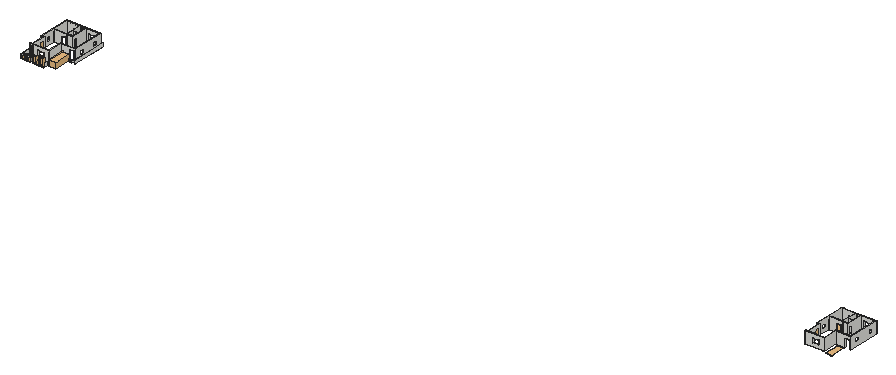
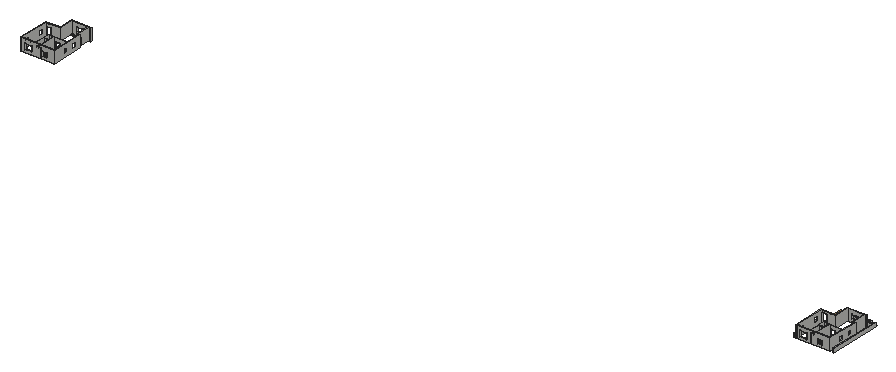
# SketchUp Ruby script. Lengths in inches.
U = 1.inch
M = Sketchup.active_model
def pt(a) = Geom::Point3d.new(a.map { |v| v * U })
def face(e, loops, mat)
  f = e.add_face(loops[0].map { |a| pt(a) })
  loops[1..].each { |l| e.add_face(l.map { |a| pt(a) }).erase! }
  f.material = f.back_material = mat if mat
  f
end
# faces: each face lists its corners as indices into pts; further lists are holes
def faces(e, pts, list, mat = nil) = list.each { |f| face(e, (f[0].is_a?(Array) ? f : [f]).map { |l| l.map { |i| pts[i] } }, mat) }
# xy, xz, yz: faces in a plane at the given z, y or x. An outline is a flat list of corners, or four numbers for a rectangle; further outlines are holes
def ring(l) = l.size == 4 ? [[l[0], l[1]], [l[2], l[1]], [l[2], l[3]], [l[0], l[3]]] : l.each_slice(2).to_a
def flat(e, list, mat, &to3) = list.each { |f| face(e, (f[0].is_a?(Array) ? f : [f]).map { |l| ring(l).map { |u, v| to3.(u, v) } }, mat) }
def xy(e, z, list, mat = nil) = flat(e, list, mat) { |x, y| [x, y, z] }
def xz(e, y, list, mat = nil) = flat(e, list, mat) { |x, z| [x, y, z] }
def yz(e, x, list, mat = nil) = flat(e, list, mat) { |y, z| [x, y, z] }
def lines(e, pts, list) = list.each { |a, b| e.add_line(pt(pts[a]), pt(pts[b])) }
# prism: a flat outline (further loops are holes) pulled along v
def prism(e, loops, v, mat = nil)
  f = face(e, loops, mat); d = Geom::Vector3d.new(v.map { |x| x * U })
  f.pushpull(f.normal.samedirection?(d) ? d.length : -d.length)
end
def box(e, o, s, mat = nil) = prism(e, [[o, [o[0] + s[0], o[1], o[2]], [o[0] + s[0], o[1] + s[1], o[2]], [o[0], o[1] + s[1], o[2]]]], [0, 0, s[2]], mat)
def at(x, y, z, deg = 0) = Geom::Transformation.translation(pt([x, y, z])) * Geom::Transformation.rotation(ORIGIN, Z_AXIS, deg.degrees)
def axes(o, x, y, z) = Geom::Transformation.new([*x, 0, *y, 0, *z, 0, *pt(o).to_a, 1])
def part(name) = M.definitions.add(name)
# library, detail: a bought-in or finely detailed component or shape, given as its bounding box
def library(name, o, s) = part(name).tap { |d| box(d.entities, o, s) }
def detail(e, o, s) = box(e.add_group.entities, o, s)
def put(e, d, t, mat = nil) = e.add_instance(d, t).tap { |i| i.material = mat if mat }
def group(e, t, mat = nil) = e.add_group.tap { |g| g.transformation = t; g.material = mat if mat }.entities
root = M.entities
M.materials.add("Rock Tiles Rough Small 19-03 250cm").color = [163, 156, 149]
M.materials.add("Wood Amboyan 13.2cm").color = [255, 255, 255]
c1 = library("Indoor Plant 004",[-26.75,-21.09,0],[44.44,41.03,87.36])
c2 = part("Component\#4")
prism(c2.entities,[[[2.98,0,0],[2.98,4,0],[2.98,4,38.3125],[2.98,24,38.3125],[2.98,24,40.375],[2.98,0,40.375]]],[-2.98,0,0],"Wood Amboyan 13.2cm")
c3 = library("Potted Plant 50-12",[-6.11,-5.26,0],[11.24,10.56,13.41])
c4 = library("Door 243 074",[-20.11,-2.41,0],[40.22,4.82,86.63])
c5 = library("Plant 260 020",[-18.86,-7.03,0.01],[33.61,20.04,67.26])
c6 = library("car",[-8.95,-10.83,0],[83.51,184.88,55.74])
c7 = part("A$C63CB6BFC")
p = [[-24,-4.5,0],[24,-4.5,0],[24,0,0],[-24,0,0],[22.01,2.25,0],[1.02,2.25,0],
  [-0.96,2.25,0],[-22.01,2.25,0],[-0.96,4.5,0],[-0.96,0,0],[1.02,0,0],[1.02,4.5,0],
  [-22.01,0,0],[-22.01,4.5,0],[22.01,0,0],[24,4.5,0],[-24,4.5,0],[22.01,4.5,0]]
lines(c7.entities,p,[[0,1],[2,3],[4,5],[6,7],[8,9],[9,10],[10,11],[3,12],[12,13],[14,2],[15,16],[15,1],
  [16,0],[17,14]])
c8 = part("new bloSDFck")
p = [[-0.99,-2.25,0],[-22.01,-2.25,0],[-0.99,-4.5,0],[-0.99,0,0],[0.99,0,0],[0.99,-4.5,0],
  [-24,-4.5,0],[-24,0,0],[-22.01,0,0],[-22.01,-4.5,0],[22.01,-4.5,0],[22.01,0,0],
  [24,0,0],[24,-4.5,0],[24,4.5,0],[-24,4.5,0],[22.01,-2.25,0],[0.99,-2.25,0]]
lines(c8.entities,p,[[0,1],[2,3],[4,5],[6,7],[7,8],[8,9],[10,11],[11,12],[12,13],[13,6],[13,14],[6,15],
  [15,14],[12,7],[16,17]])
c9 = part("FHHGGHHJ")
p = [[-7.07,-12.65,0],[-6.44,-13.01,0],[5.93,9.87,0],[5.46,10.12,0],[4.97,10.35,0],[4.49,10.58,0],
  [4,10.8,0],[3.5,11.01,0],[3,11.2,0],[2.5,11.39,0],[1.99,11.57,0],[1.48,11.74,0],
  [0.97,11.89,0],[0.45,12.04,0],[-0.07,12.18,0],[-0.59,12.3,0],[-1.11,12.42,0],[-1.64,12.52,0],
  [-2.17,12.62,0],[-2.7,12.7,0],[-3.23,12.78,0],[-3.76,12.84,0],[-4.3,12.89,0],[-4.83,12.93,0],
  [-5.37,12.96,0],[-5.91,12.98,0],[-6.44,12.99,0],[6.56,9.51,0],[8.43,8.43,0],[-6.43,-13,0],
  [-8.43,-13,0],[-8.43,-15,0],[-6.43,-15,0],[-6.43,15,0],[-8.43,15,0],[-8.43,13,0],
  [-6.43,13,0]]
lines(c9.entities,p,[[0,1],[2,3],[3,4],[4,5],[5,6],[6,7],[7,8],[8,9],[9,10],[10,11],[11,12],[12,13],
  [13,14],[14,15],[15,16],[16,17],[17,18],[18,19],[19,20],[20,21],[21,22],[22,23],[23,24],[24,25],
  [25,26],[27,28],[2,0],[27,2],[1,27],[29,30],[30,31],[31,32],[32,29],[33,34],[34,35],[35,36],
  [36,33]])
c10 = library("A$C06e6df2d",[-45.01,-35.89,0],[90.02,71.78,0.01])
c11 = part("A$C08B96C0D")
p = [[18,-10.8,0],[8,-1.8,0],[18,10.8,0],[8,1.8,0],[-18,-10.8,0],[-8,-1.8,0],
  [-18,10.8,0],[-8,1.8,0]]
lines(c11.entities,p,[[0,1],[2,3],[4,5],[6,7],[4,6],[5,7],[1,5],[3,1],[7,3],[0,4],[2,0],[6,2]])
c12 = library("STOVE-3",[-14.15,-9.8,0],[28.3,19.6,0.01])
c13 = part("dd")
p = [[-6.52,11.67,0],[-5.95,12.01,0],[5.48,-9.11,0],[5.04,-9.34,0],[4.59,-9.56,0],[4.14,-9.77,0],
  [3.6875,-9.97,0],[3.23,-10.16,0],[2.77,-10.34,0],[2.31,-10.52,0],[1.84,-10.68,0],[1.37,-10.83,0],
  [0.89,-10.98,0],[0.42,-11.11,0],[-0.0625,-11.24,0],[-0.54,-11.36,0],[-1.03,-11.46,0],[-1.51,-11.5625,0],
  [-2,-11.65,0],[-2.49,-11.73,0],[-2.98,-11.79,0],[-3.47,-11.85,0],[-3.97,-11.9,0],[-4.46,-11.9375,0],
  [-4.96,-11.97,0],[-5.45,-11.98,0],[-5.95,-11.99,0],[6.05,-8.78,0],[7.79,-7.78,0],[-5.9375,12,0],
  [-7.79,12,0],[-7.79,13.85,0],[-5.9375,13.85,0],[-5.9375,-13.85,0],[-7.79,-13.85,0],[-7.79,-12,0],
  [-5.9375,-12,0]]
lines(c13.entities,p,[[0,1],[2,3],[3,4],[4,5],[5,6],[6,7],[7,8],[8,9],[9,10],[10,11],[11,12],[12,13],
  [13,14],[14,15],[15,16],[16,17],[17,18],[18,19],[19,20],[20,21],[21,22],[22,23],[23,24],[24,25],
  [25,26],[27,28],[2,0],[27,2],[1,27],[29,30],[30,31],[31,32],[32,29],[33,34],[34,35],[35,36],
  [36,33]])
c14 = library("dasd",[-28.43,-47.8125,0],[56.86,95.625,0.01])
c15 = part("A$C1F62275E")
p = [[30,-4.5,0],[-30,-4.5,0],[-30,0,0],[30,0,0],[-28.01,2.25,0],[-0.99,2.25,0],
  [0.99,2.25,0],[28.01,2.25,0],[0.99,4.5,0],[0.99,0,0],[-0.99,0,0],[-0.99,4.5,0],
  [28.01,0,0],[28.01,4.5,0],[-28.01,4.5,0],[-28.01,0,0],[-30,4.5,0],[30,4.5,0]]
lines(c15.entities,p,[[0,1],[2,3],[4,5],[6,7],[8,9],[9,10],[10,11],[3,12],[12,13],[14,15],[15,2],[16,17],
  [16,1],[17,0]])
c16 = library("RGTE",[-11.95,-7.93,0],[23.9,15.86,0.01])
c17 = library("A$C39B3790F",[-21.92,-25.3125,0],[43.84,50.625,0.01])
c18 = library("A$C7d9d00ca",[-6.89,-10.82,0],[13.78,21.65,0.01])
c19 = library("RHG",[-21.19,-11.04,0],[42.38,22.08,0.01])
c20 = part("VEN")
p = [[-4.5,-11.98,0],[4.5,-11.98,0],[2.25,10,0],[2.25,-10,0],[0,-11.98,0],[0,11.98,0],
  [0,-10,0],[4.5,-10,0],[4.5,10,0],[0,10,0],[4.5,11.98,0],[-4.5,11.98,0]]
lines(c20.entities,p,[[0,1],[2,3],[4,5],[6,7],[8,9],[1,10],[0,11],[10,11]])
c21 = part("A$C338378D9")
p = [[-19.5,-8.5,0],[19.5,-8.5,0],[19.5,15.5,0],[-19.5,15.5,0],[-19.5,-14.5,0],[19.5,-14.5,0],
  [19.5,-9.5,0],[-19.5,-9.5,0],[-18.5,-9.5,0],[-18.5,-8.5,0],[18.5,-9.5,0],[18.5,-8.5,0],
  [-16,-15.5,0],[-17.5,-15.5,0],[-17.5,-14.5,0],[-16,-14.5,0]]
lines(c21.entities,p,[[0,1],[1,2],[2,3],[3,0],[4,5],[5,6],[6,7],[7,4],[8,9],[10,11],[12,13],[13,14],
  [14,15],[15,12]])
c22 = library("A$C0124305E",[-7.81,-9.6,0],[15.62,19.2,0.01])
c23 = library("A$C4D064DB7",[-6.63,-3.5625,0],[13.26,7.125,0.01])
c24 = library("SH",[-3.77,-3.27,-0.25],[7.54,6.54,0.5])
c25 = part("A$C231C625F")
p = [[-0.375,-18,0],[1.125,-18,0],[1.125,18,0],[-0.375,18,0],[-1.125,-27,0],[-0.375,-27,0],
  [-0.375,27,0],[-1.125,27,0]]
lines(c25.entities,p,[[0,1],[1,2],[2,3],[3,0],[4,5],[5,6],[6,7],[7,4]])
c26 = library("AC7F60799D",[-22.86,-57.6,0],[45.72,115.2,0.01])
prism(root,[[[710.23,450.625,16.75],[710.23,426.625,16.75],[710.23,426.625,23.75],[710.23,438.625,23.75],[710.23,438.625,30.75],[710.23,450.625,30.75]]],[48,0,0])
prism(root,[[[786.73,423.0625,16.75],[783.73,423.0625,16.75],[783.73,770.25,16.75],[771.73,770.25,16.75],[771.73,779.125,16.75],[786.73,779.125,16.75]]],[0,0,36])
xy(root,16.75,[[384.73,229.75,384.73,242.125,390.71,242.125,390.71,232.8125,621.84,232.8125,621.84,246.125,624.73,246.125,624.73,229.75],[621.84,246.125,621.84,248.125,394.42,248.125,394.42,266.125,624.73,266.125,624.73,246.125],[429.73,603.625,507.73,608.125],[546.73,603.625,546.73,608.125,561.73,608.125,561.73,710.125,566.23,710.125,566.23,674.125,620.23,674.125,620.23,770.125,624.73,770.125,624.73,650.125,620.23,650.125,620.23,669.625,566.23,669.625,566.23,608.125,620.23,608.125,620.23,617.125,624.73,617.125,624.73,603.625],[566.23,608.125,620.23,669.625],
  [561.73,743.125,566.23,770.125],[8197.44,814.9,8275.44,819.4],[8314.44,814.9,8314.44,819.4,8329.44,819.4,8329.44,921.4,8333.94,921.4,8333.94,885.4,8387.94,885.4,8387.94,981.4,8392.44,981.4,8392.44,861.4,8387.94,861.4,8387.94,880.9,8333.94,880.9,8333.94,819.4,8387.94,819.4,8387.94,828.4,8392.44,828.4,8392.44,814.9],[8333.94,819.4,8387.94,880.9],[8329.44,954.4,8333.94,981.4]])
xy(root,18.5625,[[384.73,229.75,624.73,229.75,624.73,246.125,621.84,246.125,621.84,232.8125,390.71,232.8125,390.71,242.125,384.73,242.125]])
xy(root,49.86,[[394.42,246.125,621.84,248.125]])
xy(root,52.75,[[394.42,246.125,624.73,266.125]])
xy(root,100.75,[[507.73,603.625,546.73,608.125],[620.23,617.125,624.73,650.125],[561.73,710.125,566.23,743.125],[8275.44,814.9,8314.44,819.4],[8387.94,828.4,8392.44,861.4],
  [8329.44,921.4,8333.94,954.4]])
xy(root,136.75,[[[429.73,603.625,624.73,603.625,624.73,770.125,620.23,770.125,620.23,674.125,566.23,674.125,566.23,770.125,561.73,770.125,561.73,608.125,429.73,608.125],[566.23,608.125,620.23,669.625]],[[8197.44,814.9,8392.44,814.9,8392.44,981.4,8387.94,981.4,8387.94,885.4,8333.94,885.4,8333.94,981.4,8329.44,981.4,8329.44,819.4,8197.44,819.4],[8333.94,819.4,8387.94,880.9]]])
xz(root,229.75,[[384.73,16.75,624.73,18.5625]])
xz(root,232.8125,[[390.71,16.75,621.84,18.5625]])
xz(root,242.125,[[384.73,16.75,390.71,18.5625]])
xz(root,246.125,[[621.84,16.75,624.73,18.5625],[621.84,18.5625,624.73,18.5625,624.73,52.75,394.42,52.75,394.42,49.86,621.84,49.86]])
xz(root,248.125,[[394.42,16.75,621.84,49.86]],"Rock Tiles Rough Small 19-03 250cm")
xz(root,266.125,[[394.42,16.75,624.73,52.75]])
xz(root,603.625,[[429.73,16.75,507.73,16.75,507.73,100.75,546.73,100.75,546.73,16.75,624.73,16.75,624.73,136.75,429.73,136.75]])
xz(root,608.125,[[429.73,16.75,429.73,136.75,561.73,136.75,561.73,16.75,546.73,16.75,546.73,100.75,507.73,100.75,507.73,16.75],[566.23,16.75,620.23,136.75]])
xz(root,617.125,[[620.23,16.75,624.73,100.75]])
xz(root,650.125,[[620.23,16.75,624.73,100.75]])
xz(root,669.625,[[566.23,16.75,620.23,136.75]])
xz(root,674.125,[[566.23,16.75,620.23,136.75]])
xz(root,710.125,[[561.73,16.75,566.23,100.75]])
xz(root,743.125,[[561.73,16.75,566.23,100.75]])
xz(root,770.125,[[561.73,16.75,566.23,136.75],[620.23,16.75,624.73,136.75]])
xz(root,814.9,[[8197.44,16.75,8275.44,16.75,8275.44,100.75,8314.44,100.75,8314.44,16.75,8392.44,16.75,8392.44,136.75,8197.44,136.75]])
xz(root,819.4,[[8197.44,16.75,8197.44,136.75,8329.44,136.75,8329.44,16.75,8314.44,16.75,8314.44,100.75,8275.44,100.75,8275.44,16.75],[8333.94,16.75,8387.94,136.75]])
xz(root,828.4,[[8387.94,16.75,8392.44,100.75]])
xz(root,861.4,[[8387.94,16.75,8392.44,100.75]])
xz(root,880.9,[[8333.94,16.75,8387.94,136.75]])
xz(root,885.4,[[8333.94,16.75,8387.94,136.75]])
xz(root,921.4,[[8329.44,16.75,8333.94,100.75]])
xz(root,954.4,[[8329.44,16.75,8333.94,100.75]])
xz(root,981.4,[[8329.44,16.75,8333.94,136.75],[8387.94,16.75,8392.44,136.75]])
yz(root,384.73,[[229.75,16.75,242.125,18.5625]])
yz(root,390.71,[[232.8125,16.75,242.125,18.5625]])
yz(root,394.42,[[248.125,16.75,248.125,49.86,246.125,49.86,246.125,52.75,266.125,52.75,266.125,16.75]])
yz(root,429.73,[[603.625,16.75,608.125,136.75]])
yz(root,507.73,[[603.625,16.75,608.125,100.75]])
yz(root,546.73,[[603.625,16.75,608.125,100.75]])
yz(root,561.73,[[608.125,16.75,608.125,136.75,770.125,136.75,770.125,16.75,743.125,16.75,743.125,100.75,710.125,100.75,710.125,16.75]])
yz(root,566.23,[[608.125,16.75,669.625,136.75],[674.125,16.75,710.125,16.75,710.125,100.75,743.125,100.75,743.125,16.75,770.125,16.75,770.125,136.75,674.125,136.75]])
yz(root,620.23,[[608.125,16.75,608.125,136.75,669.625,136.75,669.625,16.75,650.125,16.75,650.125,100.75,617.125,100.75,617.125,16.75],[674.125,16.75,770.125,136.75]])
yz(root,621.84,[[232.8125,16.75,246.125,18.5625],[246.125,16.75,248.125,49.86]])
yz(root,624.73,[[229.75,16.75,246.125,18.5625],[246.125,16.75,266.125,52.75],[603.625,16.75,617.125,16.75,617.125,100.75,650.125,100.75,650.125,16.75,770.125,16.75,770.125,136.75,603.625,136.75]])
yz(root,8197.44,[[814.9,16.75,819.4,136.75]])
yz(root,8275.44,[[814.9,16.75,819.4,100.75]])
yz(root,8314.44,[[814.9,16.75,819.4,100.75]])
yz(root,8329.44,[[819.4,16.75,819.4,136.75,981.4,136.75,981.4,16.75,954.4,16.75,954.4,100.75,921.4,100.75,921.4,16.75]])
yz(root,8333.94,[[819.4,16.75,880.9,136.75],[885.4,16.75,921.4,16.75,921.4,100.75,954.4,100.75,954.4,16.75,981.4,16.75,981.4,136.75,885.4,136.75]])
yz(root,8387.94,[[819.4,16.75,819.4,136.75,880.9,136.75,880.9,16.75,861.4,16.75,861.4,100.75,828.4,100.75,828.4,16.75],[885.4,16.75,981.4,136.75]])
yz(root,8392.44,[[814.9,16.75,828.4,16.75,828.4,100.75,861.4,100.75,861.4,16.75,981.4,16.75,981.4,136.75,814.9,136.75]])
g1 = group(root,at(384.73,242.125,16.75))
box(g1,[0,0,0],[9.6875,537,36])
put(root,c1,axes([399.61,242.54,16.75],[0.28,0,0],[0,0.28,0],[0,0,0.28]))
put(root,c2,at(420.99,242.125,16.75),"Wood Amboyan 13.2cm")
put(root,c2,at(425.47,242.125,16.75))
put(root,c2,at(429.95,242.125,16.75))
put(root,c3,at(434.3125,237.77,16.75))
put(root,c2,at(434.4375,242.125,16.75))
put(root,c2,at(438.92,242.125,16.75))
put(root,c2,at(443.4,242.125,16.75))
put(root,c4,axes([448.64,419.125,16.75],[0,-0.82032,0],[1,0,0],[0,0,0.9696]))
put(root,c2,at(447.88,242.125,16.75))
put(root,c2,at(452.37,242.125,16.75))
put(root,c3,at(456.52,237.24,16.75))
put(root,c1,axes([462.74,242.54,16.75],[0.28,0,0],[0,0.28,0],[0,0,0.28]))
put(root,c5,at(527.48,240.83,16.75))
put(root,c1,axes([547.8,242.54,16.75],[0.28,0,0],[0,0.28,0],[0,0,0.28]))
put(root,c3,at(571.5625,239.98,16.75))
put(root,c3,at(582.87,241.41,16.75))
put(root,c5,at(596.17,242.31,16.75))
g2 = group(root,at(420.73,287.125,16.75))
xy(g2,0,[[0,15,0,24,21,24,21,115.5,30,115.5,30,24,195,24,195,172.5,289.5,172.5,289.5,163.5,204,163.5,204,15],[21,148.5,21,163.5,0,163.5,0,483,9,483,9,172.5,30,172.5,30,148.5],[337.5,163.5,337.5,172.5,342,172.5,342,492,351,492,351,163.5],[0,483,342,492]])
xy(g2,24,[[78,483,126,492],[234,483,306,492]])
xy(g2,36,[[86,15,146,24],[0,220.5,9,268.5],[342,220.5,351,268.5],[0,331.84,9,379.84],[342,391.58,351,439.58]])
xy(g2,72,[[78,483,126,492]])
xy(g2,84,[[86,15,146,24],[21,115.5,30,148.5],[0,220.5,9,268.5],[342,220.5,351,268.5],[0,331.84,9,379.84],
  [342,391.58,351,439.58],[234,483,306,492]])
xy(g2,90,[[160.6,483,184.56,492]])
xy(g2,98,[[289.5,163.5,337.5,172.5]])
xy(g2,108,[[160.6,483,184.56,492]])
xy(g2,120,[[0,15,204,15,204,163.5,351,163.5,351,492,342,492,342,172.5,195,172.5,195,24,30,24,30,172.5,9,172.5,9,483,0,483,0,163.5,21,163.5,21,24,0,24],[0,483,342,492]])
xz(g2,15,[[[0,0,204,120],[86,36,146,84]]])
xz(g2,24,[[0,0,21,120],[[30,0,195,120],[86,36,146,84]]])
xz(g2,115.5,[[21,0,30,84]])
xz(g2,148.5,[[21,0,30,84]])
xz(g2,163.5,[[0,0,21,120],[204,0,289.5,0,289.5,98,337.5,98,337.5,0,351,0,351,120,204,120]])
xz(g2,172.5,[[9,0,30,120],[195,0,195,120,342,120,342,0,337.5,0,337.5,98,289.5,98,289.5,0]])
xz(g2,220.5,[[0,36,9,84],[342,36,351,84]])
xz(g2,268.5,[[0,36,9,84],[342,36,351,84]])
xz(g2,331.84,[[0,36,9,84]])
xz(g2,379.84,[[0,36,9,84]])
xz(g2,391.58,[[342,36,351,84]])
xz(g2,439.58,[[342,36,351,84]])
xz(g2,483,[[[9,0,342,120],[234,24,306,84],[78,24,126,72],[160.6,90,184.56,108]]])
xz(g2,492,[[[0,0,351,120],[234,24,306,84],[78,24,126,72],[160.6,90,184.56,108]]])
yz(g2,0,[[15,0,24,120],[[163.5,0,492,120],[331.84,36,379.84,84],[220.5,36,268.5,84]]])
yz(g2,9,[[[172.5,0,483,120],[331.84,36,379.84,84],[220.5,36,268.5,84]]])
yz(g2,21,[[24,0,24,120,163.5,120,163.5,0,148.5,0,148.5,84,115.5,84,115.5,0]])
yz(g2,30,[[24,0,115.5,0,115.5,84,148.5,84,148.5,0,172.5,0,172.5,120,24,120]])
yz(g2,78,[[483,24,492,72]])
yz(g2,86,[[15,36,24,84]])
yz(g2,126,[[483,24,492,72]])
yz(g2,146,[[15,36,24,84]])
yz(g2,160.6,[[483,90,492,108]])
yz(g2,184.56,[[483,90,492,108]])
yz(g2,195,[[24,0,172.5,120]])
yz(g2,204,[[15,0,163.5,120]])
yz(g2,234,[[483,24,492,84]])
yz(g2,289.5,[[163.5,0,172.5,98]])
yz(g2,306,[[483,24,492,84]])
yz(g2,337.5,[[163.5,0,172.5,98]])
yz(g2,342,[[[172.5,0,483,120],[220.5,36,268.5,84],[391.58,36,439.58,84]]])
yz(g2,351,[[[163.5,0,492,120],[220.5,36,268.5,84],[391.58,36,439.58,84]]])
# 2 loose lines left out
put(root,c6,axes([648.64,283.75,16.75],[0.82,0,0],[0,1,0],[0,0,1]))
put(root,c7,axes([8192.94,854.24,16.75],[0,1,0],[1,0,0],[0,0,1]))
put(root,c8,at(8192.94,742.9,16.75,90))
put(root,c4,axes([8216.35,630.4,16.75],[0,-0.82032,0],[1,0,0],[0,0,0.9696]))
put(root,c9,axes([8218.72,630.4,16.75],[1.1,0,0],[0,-1.1,0],[0,0,1.1]))
put(root,c10,at(8233.9375,886.8125,16.75,-90))
put(root,c11,axes([8259.76,534.9,16.75],[1,0,0],[0,-1,0],[0,0,1]))
put(root,c12,axes([8259.91,535.56,16.75],[-1,0,0],[0,1,0],[0,0,1]))
put(root,c7,axes([8290.44,985.9,16.75],[1,0,0],[0,-1,0],[0,0,1]))
put(root,c13,axes([8294.94,825.87,16.75],[0,1.40833,0],[1.40833,0,0],[0,0,1.40833]))
put(root,c14,at(8301.07,749.56,16.75,-90))
put(root,c15,at(8304.45,517.9,16.75))
put(root,c16,axes([8319.375,973.02,16.75],[-0.86556,0.2466,0],[-0.2466,-0.86556,0],[0,0,0.9]))
put(root,c9,axes([8338.72,937.9,16.75],[1.1,0,0],[0,1.1,0],[0,0,1.1]))
put(root,c17,axes([8339.96,825.4,16.75],[-0.2514,-0.2514,0],[0.2514,-0.2514,0],[0,0,0.35554]))
put(root,c18,axes([8344.77,862.9,16.75],[0,-1,0],[-1,0,0],[0,0,1]))
put(root,c19,axes([8359.25,533.44,16.75],[1,0,0],[0,-1,0],[0,0,1]))
put(root,c20,at(8361.02,985.9,16.75,-90))
g3 = group(root,at(8188.44,498.4,16.75))
xy(g3,0,[[0,15,0,24,21,24,21,115.5,30,115.5,30,24,195,24,195,172.5,289.5,172.5,289.5,163.5,204,163.5,204,15],[21,148.5,21,163.5,0,163.5,0,483,9,483,9,172.5,30,172.5,30,148.5],[337.5,163.5,337.5,172.5,342,172.5,342,492,351,492,351,163.5],[0,483,342,492]])
xy(g3,24,[[78,483,126,492],[234,483,306,492]])
xy(g3,36,[[86,15,146,24],[0,220.5,9,268.5],[342,220.5,351,268.5],[0,331.84,9,379.84],[342,391.58,351,439.58]])
xy(g3,72,[[78,483,126,492]])
xy(g3,84,[[86,15,146,24],[21,115.5,30,148.5],[289.5,163.5,337.5,172.5],[0,220.5,9,268.5],[342,220.5,351,268.5],
  [0,331.84,9,379.84],[342,391.58,351,439.58],[234,483,306,492]])
xy(g3,90,[[160.6,483,184.56,492]])
xy(g3,108,[[160.6,483,184.56,492]])
xy(g3,120,[[0,15,204,15,204,163.5,351,163.5,351,492,342,492,342,172.5,195,172.5,195,24,30,24,30,172.5,9,172.5,9,483,0,483,0,163.5,21,163.5,21,24,0,24],[0,483,342,492]])
xz(g3,15,[[[0,0,204,120],[86,36,146,84]]])
xz(g3,24,[[0,0,21,120],[[30,0,195,120],[86,36,146,84]]])
xz(g3,115.5,[[21,0,30,84]])
xz(g3,148.5,[[21,0,30,84]])
xz(g3,163.5,[[0,0,21,120],[204,0,289.5,0,289.5,84,337.5,84,337.5,0,351,0,351,120,204,120]])
xz(g3,172.5,[[9,0,30,120],[195,0,195,120,342,120,342,0,337.5,0,337.5,84,289.5,84,289.5,0]])
xz(g3,220.5,[[0,36,9,84],[342,36,351,84]])
xz(g3,268.5,[[0,36,9,84],[342,36,351,84]])
xz(g3,331.84,[[0,36,9,84]])
xz(g3,379.84,[[0,36,9,84]])
xz(g3,391.58,[[342,36,351,84]])
xz(g3,439.58,[[342,36,351,84]])
xz(g3,483,[[[9,0,342,120],[234,24,306,84],[78,24,126,72],[160.6,90,184.56,108]]])
xz(g3,492,[[[0,0,351,120],[234,24,306,84],[78,24,126,72],[160.6,90,184.56,108]]])
yz(g3,0,[[15,0,24,120],[[163.5,0,492,120],[331.84,36,379.84,84],[220.5,36,268.5,84]]])
yz(g3,9,[[[172.5,0,483,120],[331.84,36,379.84,84],[220.5,36,268.5,84]]])
yz(g3,21,[[24,0,24,120,163.5,120,163.5,0,148.5,0,148.5,84,115.5,84,115.5,0]])
yz(g3,30,[[24,0,115.5,0,115.5,84,148.5,84,148.5,0,172.5,0,172.5,120,24,120]])
yz(g3,78,[[483,24,492,72]])
yz(g3,86,[[15,36,24,84]])
yz(g3,126,[[483,24,492,72]])
yz(g3,146,[[15,36,24,84]])
yz(g3,160.6,[[483,90,492,108]])
yz(g3,184.56,[[483,90,492,108]])
yz(g3,195,[[24,0,172.5,120]])
yz(g3,204,[[15,0,163.5,120]])
yz(g3,234,[[483,24,492,84]])
yz(g3,289.5,[[163.5,0,172.5,84]])
yz(g3,306,[[483,24,492,84]])
yz(g3,337.5,[[163.5,0,172.5,84]])
yz(g3,342,[[[172.5,0,483,120],[220.5,36,268.5,84],[391.58,36,439.58,84]]])
yz(g3,351,[[[163.5,0,492,120],[220.5,36,268.5,84],[391.58,36,439.58,84]]])
# 5 loose lines left out
put(root,c21,axes([8371.7,595.93,16.75],[0,-0.69231,0],[0.69231,0,0],[0,0,0.69231]))
put(root,c18,at(8377.12,963.4,16.75,-90))
put(root,c22,at(8380.14,933.87,16.75))
put(root,c23,axes([8381.31,903.21,16.75],[1,0,0],[0,-1,0],[0,0,1]))
put(root,c9,axes([8383.17,844.9,16.75],[-1.1,0,0],[0,1.1,0],[0,0,1.1]))
put(root,c24,axes([8384.67,903.18,17],[0,1.00172,0],[1.00172,0,0],[0,0,1.00172]))
put(root,c25,axes([8393.57,922.82,16.75],[-1,0,0],[0,1,0],[0,0,1]))
put(root,c26,axes([8448.66,571.97,16.75],[-1.35844,0,0],[0,1.35844,0],[0,0,1.35844]))
